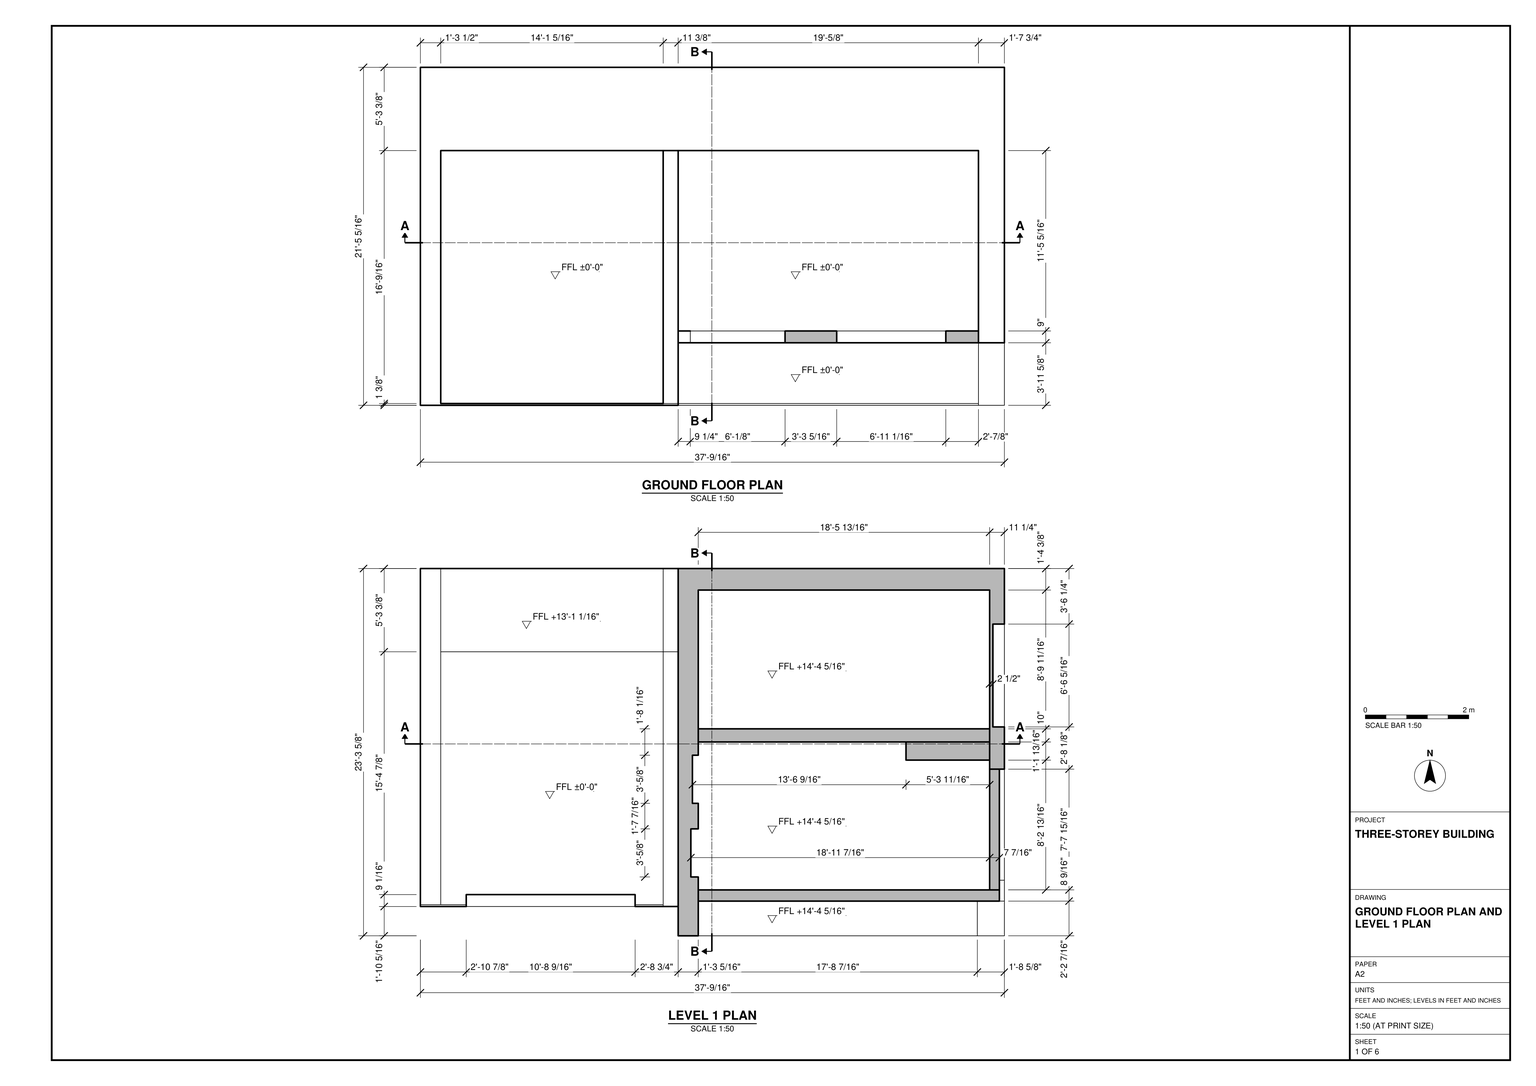
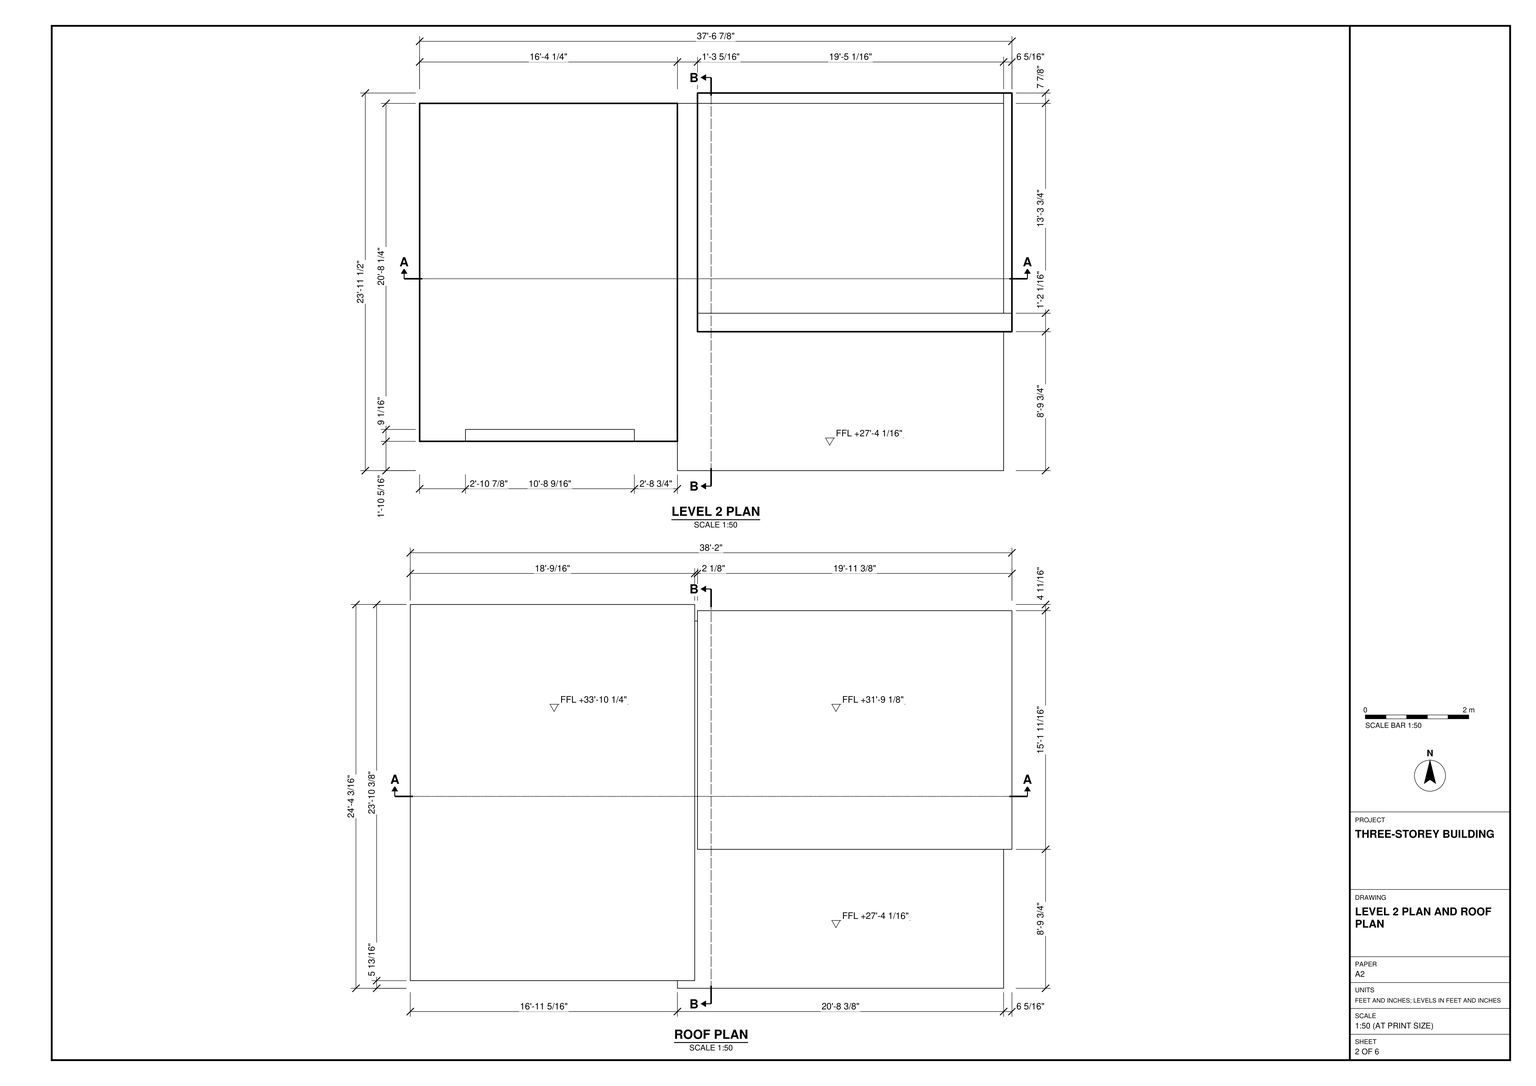
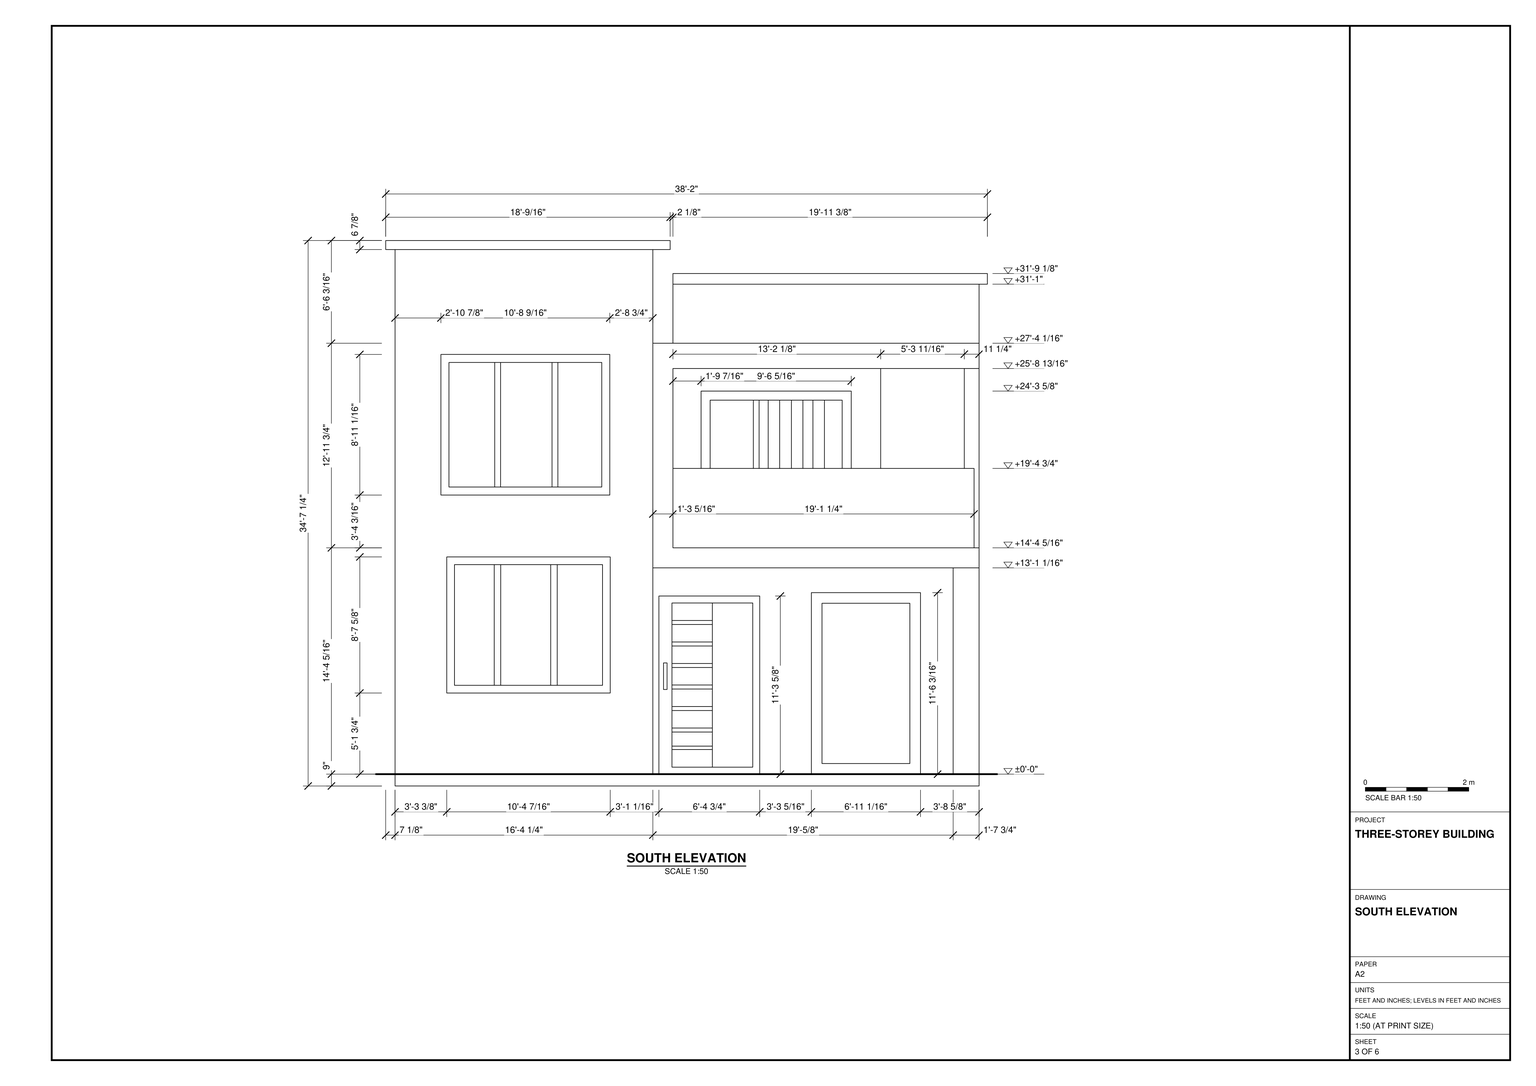
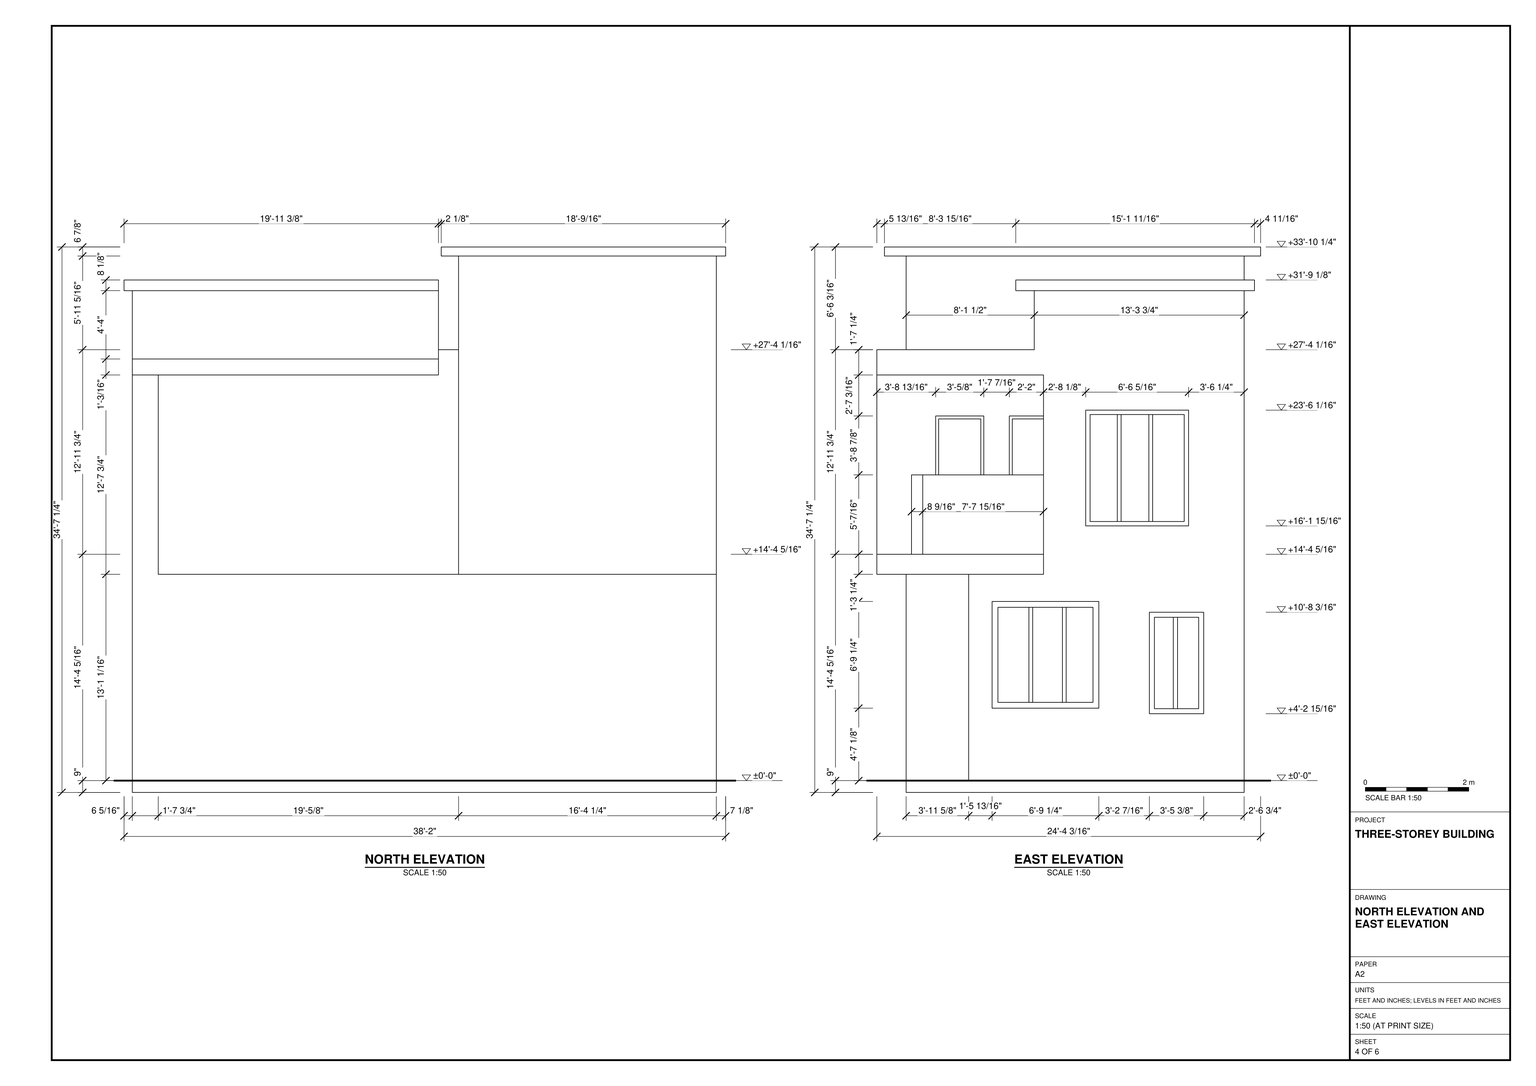
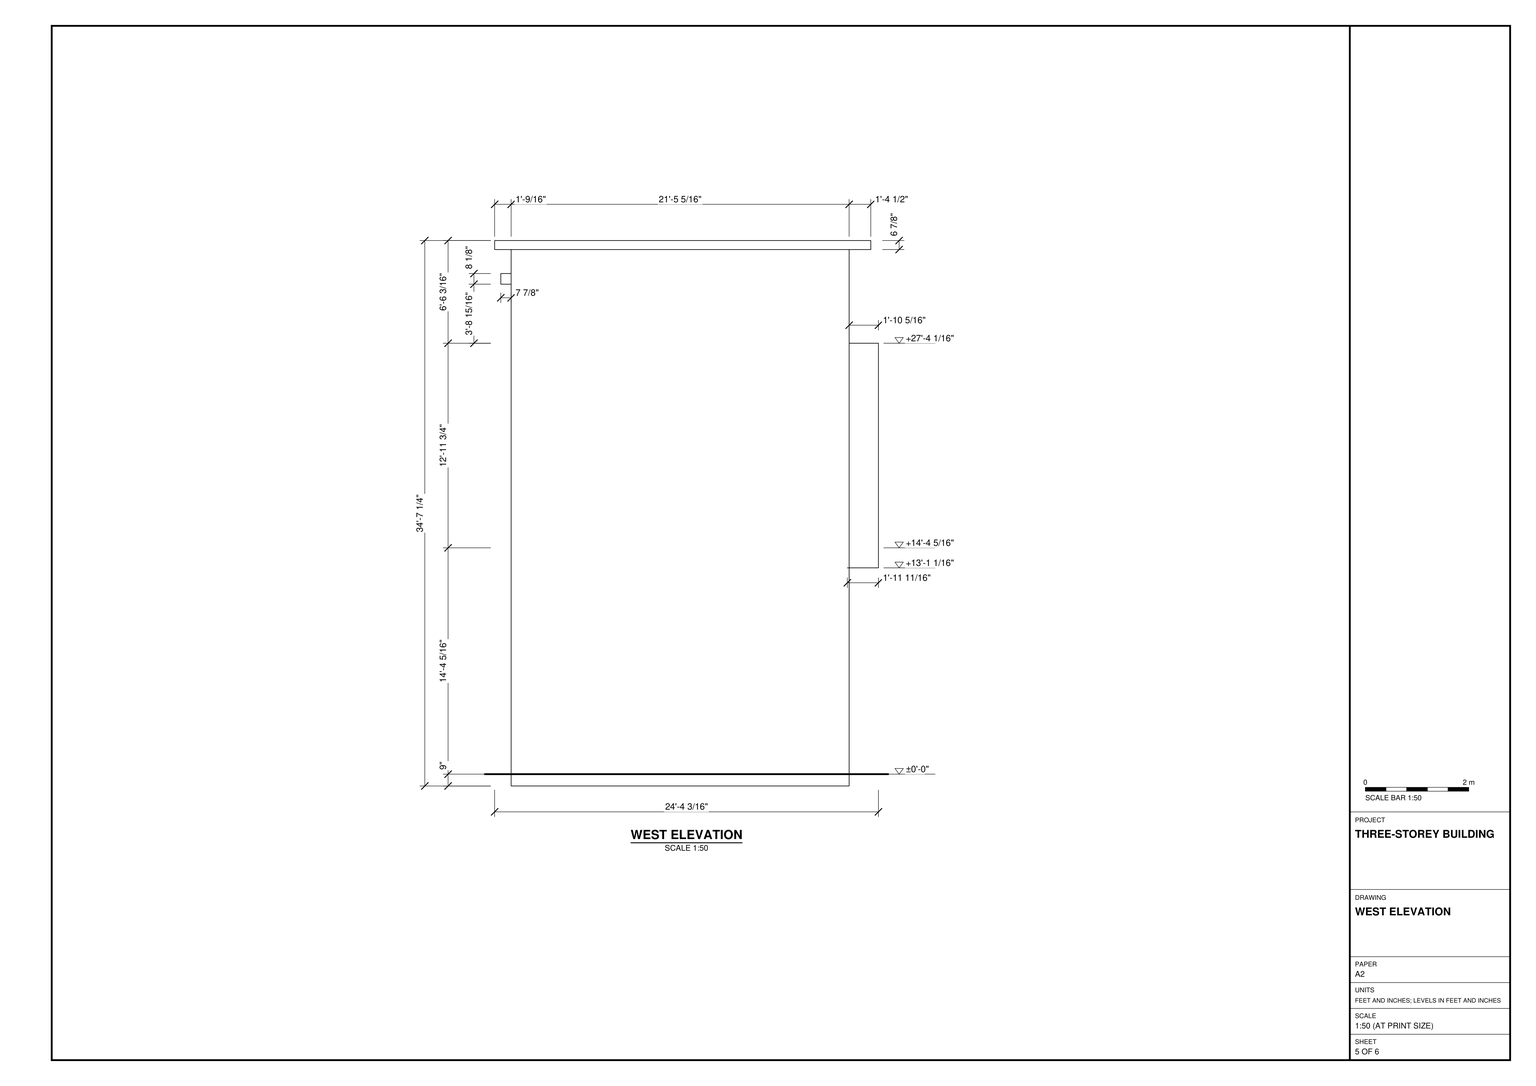
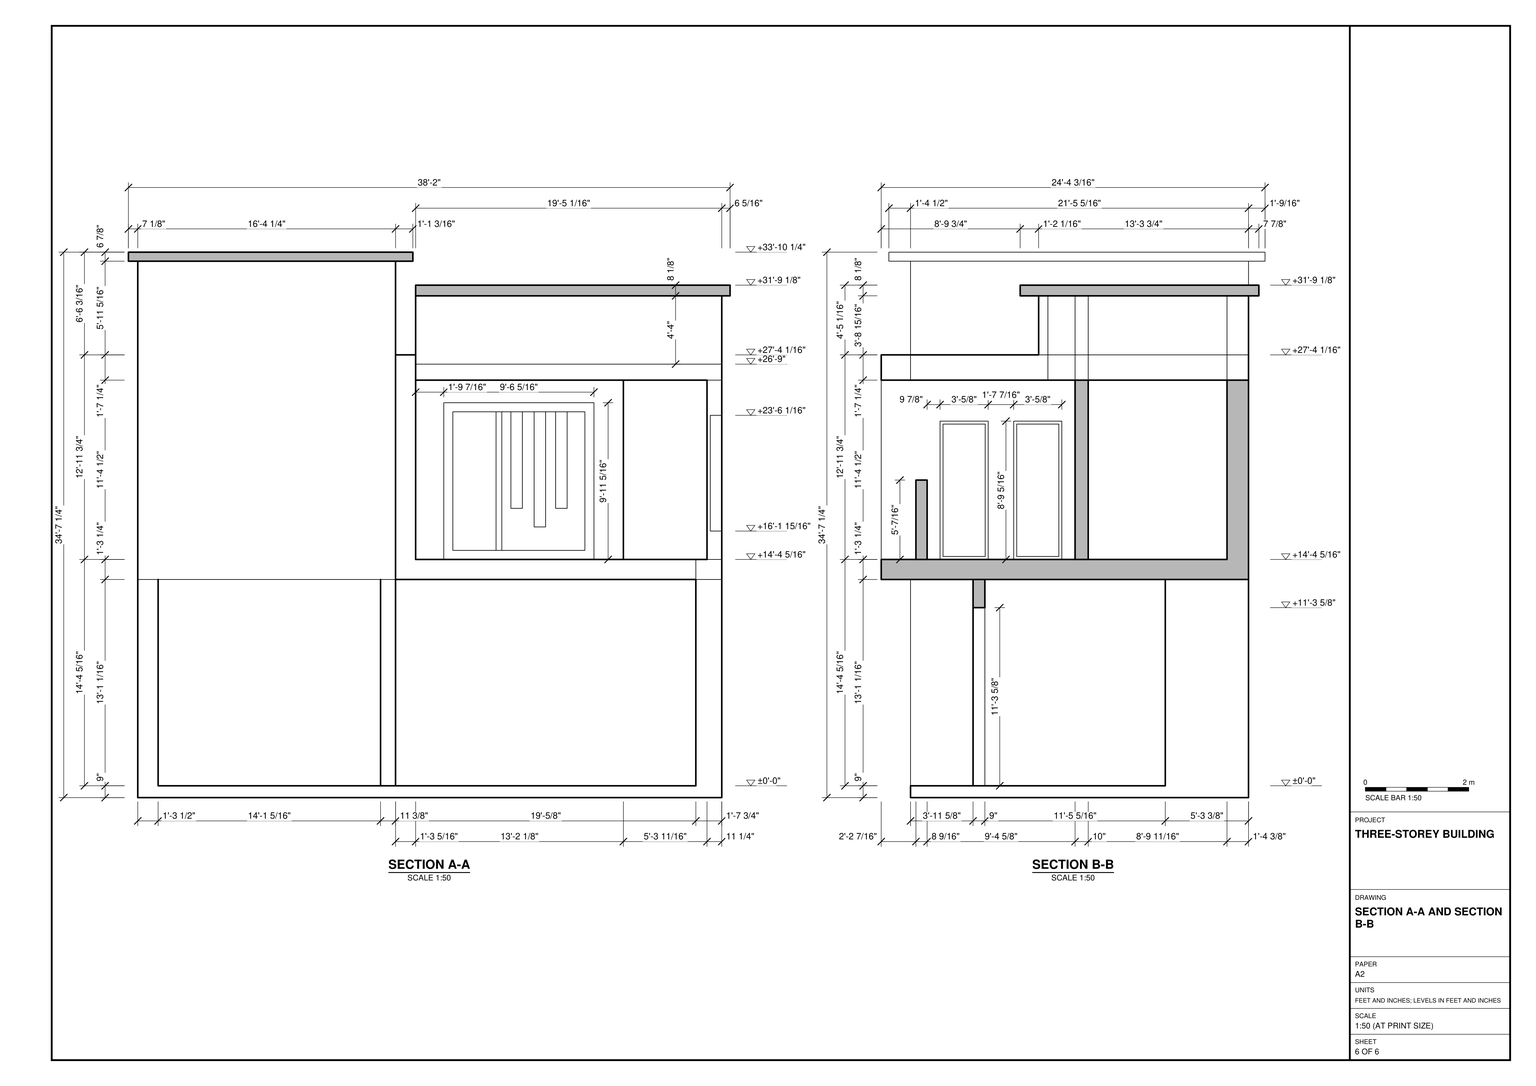
Build the three-storey building in SketchUp using task_files/diagram_01.pdf. Work in feet and inches. The overall model extents are 38'-2" along X, 24'-4 3/16" along Y and 34'-7 1/4" along Z. Set the ground floor at ±0'-0", Level 1 at +14'-4 5/16" and Level 2 at +27'-4 1/16".

Lay out the two adjoining bays from the plans. Follow the wall thicknesses, returns and slab outlines at each level, keeping the area marked at ground-floor level on the Level 1 plan open above. Use the south elevation to place the stacked window units in the taller bay and the entrance door and adjacent tall opening in the other bay. Model the recessed balcony above the entrance, including its solid front and the framed opening behind it. Match the separate flat roof slabs to their respective footprints and heights, leaving the front part of Level 2 exposed as drawn. Include stairs, built-in joinery and main furniture only where shown.

Keep walls, slabs, roofs and each furniture or joinery piece in separate groups or components, and use components for repeated parts. Decor and loose items may be any suitable library components. Save one SketchUp model as output_files/three_storey_building_with_recessed_balcony.skp.

# SketchUp Ruby script. Lengths in inches.
U = 1.inch
M = Sketchup.active_model
def pt(a) = Geom::Point3d.new(a.map { |v| v * U })
def face(e, loops, mat)
  f = e.add_face(loops[0].map { |a| pt(a) })
  loops[1..].each { |l| e.add_face(l.map { |a| pt(a) }).erase! }
  f.material = f.back_material = mat if mat
  f
end
# faces: each face lists its corners as indices into pts; further lists are holes
def faces(e, pts, list, mat = nil) = list.each { |f| face(e, (f[0].is_a?(Array) ? f : [f]).map { |l| l.map { |i| pts[i] } }, mat) }
# xy, xz, yz: faces in a plane at the given z, y or x. An outline is a flat list of corners, or four numbers for a rectangle; further outlines are holes
def ring(l) = l.size == 4 ? [[l[0], l[1]], [l[2], l[1]], [l[2], l[3]], [l[0], l[3]]] : l.each_slice(2).to_a
def flat(e, list, mat, &to3) = list.each { |f| face(e, (f[0].is_a?(Array) ? f : [f]).map { |l| ring(l).map { |u, v| to3.(u, v) } }, mat) }
def xy(e, z, list, mat = nil) = flat(e, list, mat) { |x, y| [x, y, z] }
def xz(e, y, list, mat = nil) = flat(e, list, mat) { |x, z| [x, y, z] }
def yz(e, x, list, mat = nil) = flat(e, list, mat) { |y, z| [x, y, z] }
def lines(e, pts, list) = list.each { |a, b| e.add_line(pt(pts[a]), pt(pts[b])) }
# prism: a flat outline (further loops are holes) pulled along v
def prism(e, loops, v, mat = nil)
  f = face(e, loops, mat); d = Geom::Vector3d.new(v.map { |x| x * U })
  f.pushpull(f.normal.samedirection?(d) ? d.length : -d.length)
end
def box(e, o, s, mat = nil) = prism(e, [[o, [o[0] + s[0], o[1], o[2]], [o[0] + s[0], o[1] + s[1], o[2]], [o[0], o[1] + s[1], o[2]]]], [0, 0, s[2]], mat)
def at(x, y, z, deg = 0) = Geom::Transformation.translation(pt([x, y, z])) * Geom::Transformation.rotation(ORIGIN, Z_AXIS, deg.degrees)
def axes(o, x, y, z) = Geom::Transformation.new([*x, 0, *y, 0, *z, 0, *pt(o).to_a, 1])
def part(name) = M.definitions.add(name)
# library, detail: a bought-in or finely detailed component or shape, given as its bounding box
def library(name, o, s) = part(name).tap { |d| box(d.entities, o, s) }
def detail(e, o, s) = box(e.add_group.entities, o, s)
def put(e, d, t, mat = nil) = e.add_instance(d, t).tap { |i| i.material = mat if mat }
def group(e, t, mat = nil) = e.add_group.tap { |g| g.transformation = t; g.material = mat if mat }.entities
root = M.entities
M.materials.add("[Formica Beige]").color = [211, 187, 149]
M.materials.add("[Formica Laminate Dark]").color = [50, 53, 60]
M.materials.add("[Formica Laminate Light]").color = [213, 189, 164]
M.materials.add("[Formica Speckled Grey]").color = [56, 62, 66]
M.materials.add("[Formica Speckled Grey]1").color = [94, 105, 111]
M.materials.add("[Quartz Light Brown]").color = [199, 184, 152]
M.materials.add("[Translucent Glass Gray]").color = [128, 128, 128]
M.materials["[Translucent Glass Gray]"].alpha = 0.5
M.materials.add("[Translucent Glass Safety]").color = [204, 235, 244]
M.materials["[Translucent Glass Safety]"].alpha = 0.5
M.materials.add("[Wood Floor Dark]").color = [153, 94, 42]
M.materials.add("[Wood Floor Light]").color = [204, 176, 127]
M.materials.add("[Wood Floor Parquet]").color = [81, 50, 21]
M.materials.add("[Wood Floor]").color = [91, 62, 36]
M.materials.add("[Wood Veneer 01]").color = [84, 49, 25]
M.materials.add("[Wood Veneer 01]1").color = [120, 70, 37]
xy(root,0,[[7.125,22.3125,451.7,279.61]])
xy(root,9,[[203.35,22.3125,431.96,23.68],[431.96,22.3125,451.7,69.91],[22.61,23.68,191.94,216.24],[191.94,23.68,203.35,216.24],[203.35,23.68,431.96,69.91],
  [203.35,69.91,212.59,78.9],[212.59,69.91,284.72,78.9],[284.72,69.91,324.04,78.9],[324.04,69.91,407.1,78.9],[407.1,69.91,431.96,78.9],
  [203.35,78.9,431.96,216.24]])
xy(root,144.625,[[212.59,69.91,284.72,78.9]])
xy(root,147.1875,[[324.04,69.91,407.1,78.9]])
xy(root,166.0625,[[203.35,0,451.7,69.91],[203.35,69.91,431.96,78.9],[431.96,69.91,451.7,78.9],[203.35,78.9,431.96,216.24],[22.61,216.24,191.94,279.61],
  [191.94,216.24,203.35,279.61],[203.35,216.24,431.96,279.61]])
xy(root,181.3125,[[218.65,0,431.09,26.41],[431.09,0,451.7,26.41],[218.65,26.41,431.09,34.95],[431.09,26.41,447.9,34.95],[447.9,26.41,451.7,42.31],
  [218.65,34.95,440.46,34.95,440.46,133.76,376.8,133.76,376.8,147.57,218.65,147.57,218.65,137.48,214.21,137.48,214.21,100.85,218.65,100.85,218.65,81.42,213.02,81.42,213.02,44.79,218.65,44.79],[440.46,34.95,447.9,126.88],[447.9,42.31,451.7,126.88],[376.8,133.76,431.96,147.57],[431.96,133.76,440.46,147.57],
  [218.65,147.57,440.46,157.57],[218.65,157.57,440.46,263.23]])
xy(root,202.92,[[442.95,159.01,451.7,237.33]])
xy(root,221.48,[[42.02,22.3125,170.58,31.375]])
xy(root,241.75,[[218.65,26.41,447.9,34.95],[440.46,34.95,447.9,126.88]],"[Translucent Glass Safety]")
xy(root,286.625,[[213.02,44.79,218.65,81.42],[214.21,100.85,218.65,137.48]])
xy(root,291.04,[[442.95,159.01,451.7,237.33]])
xy(root,317.8125,[[218.65,0,218.65,147.57,376.8,147.57,376.8,133.76,440.46,133.76,440.46,0],[440.46,0,451.7,126.88],[376.8,133.76,440.46,147.57],[218.65,147.57,440.46,157.57],[218.65,157.57,440.46,263.23],
  [218.65,263.23,440.46,279.61]])
xy(root,328.54,[[42.02,22.3125,170.58,31.375]])
xy(root,337.0625,[[203.35,0,451.7,0,451.7,119.84,218.65,119.84,218.65,279.61,203.35,279.61]])
xy(root,382,[[218.65,105.77,458.01,119.84],[218.65,119.84,451.7,279.61],[451.7,119.84,458.01,287.48],[218.65,279.61,451.7,287.48]])
xy(root,390.125,[[218.65,105.77,458.01,287.48]])
xy(root,408.375,[[7.125,22.3125,203.35,279.61],[7.125,279.61,203.35,292.17]])
xy(root,408.375,[[0,5.8125,216.53,22.3125],[0,22.3125,7.125,292.17],[203.35,22.3125,216.53,292.17]],"[Formica Speckled Grey]1")
xy(root,415.25,[[0,5.8125,216.53,292.17]])
xz(root,0,[[203.35,166.0625,451.7,166.0625,451.7,181.3125,218.65,181.3125,218.65,317.8125,451.7,317.8125,451.7,337.0625,203.35,337.0625]])
xz(root,5.8125,[[0,408.375,216.53,415.25]])
xz(root,22.3125,[[[7.125,0,451.7,0,451.7,9,203.35,9,203.35,408.375,7.125,408.375],[42.02,221.48,170.58,328.54],[46.48,70.76,170.92,174.38]]])
xz(root,22.3125,[[[46.48,70.76,170.92,174.38],[52.35,76.63,165.05,168.52]],[82.61,76.63,87.56,168.52],[125.61,76.63,130.56,168.52]],"[Formica Speckled Grey]")
xz(root,22.3125,[[52.35,76.63,82.61,168.52],[87.56,76.63,125.61,168.52],[130.56,76.63,165.05,168.52]],"[Translucent Glass Safety]")
xz(root,23.68,[[22.61,9,191.94,166.0625]])
xz(root,26.41,[[218.65,181.3125,447.9,241.75]],"[Translucent Glass Safety]")
xz(root,31.375,[[[42.02,221.48,170.58,328.54],[48.14,227.6,164.46,322.42]],[82.98,227.6,87.4375,322.42],[126.6,227.6,131.0625,322.42]],"[Formica Speckled Grey]")
xz(root,31.375,[[48.14,227.6,82.98,322.42],[87.4375,227.6,126.6,322.42],[131.0625,227.6,164.46,322.42]],"[Translucent Glass Safety]")
xz(root,34.95,[[431.09,181.3125,440.46,241.75],[440.46,181.3125,447.9,241.75]])
xz(root,34.95,[[218.65,181.3125,431.09,241.75]],"[Translucent Glass Safety]")
xz(root,44.79,[[213.02,181.3125,218.65,286.625]])
xz(root,69.91,[[203.35,9,207.97,9,207.97,144.625,284.72,144.625,284.72,9,324.04,9,324.04,147.1875,407.1,147.1875,407.1,9,431.96,9,431.96,166.0625,203.35,166.0625],[431.96,9,451.7,166.0625]])
xz(root,69.91,[[211.49,73.44,214.17,93.69]],"[Formica Beige]")
xz(root,69.91,[[217.9,27.75,248.65,30.33],[217.9,41.0625,248.65,44.12],[217.9,57.4375,248.65,60.5],[217.9,73.8125,248.65,76.87],[217.9,90.1875,248.65,93.25],
  [217.9,106.5625,248.65,109.62],[217.9,122.9375,248.65,126]],"[Quartz Light Brown]")
xz(root,69.91,[[332.125,17.09,399.01,139.1]],"[Translucent Glass Gray]")
xz(root,69.91,[[248.65,14.3125,279.41,139.3125]],"[Translucent Glass Safety]")
xz(root,69.91,[[217.9,14.3125,248.65,27.75],[217.9,30.33,248.65,41.0625],[217.9,44.12,248.65,57.4375],[217.9,60.5,248.65,73.8125],[217.9,76.87,248.65,90.1875],
  [217.9,93.25,248.65,106.5625],[217.9,109.62,248.65,122.9375],[217.9,126,248.65,139.3125]],"[Wood Floor Dark]")
xz(root,69.91,[[[207.97,9,284.72,144.625],[217.9,14.3125,279.41,139.3125],[211.49,73.44,214.17,93.69]]],"[Wood Floor Parquet]")
xz(root,69.91,[[[324.04,9,407.1,147.1875],[332.125,17.09,399.01,139.1]]],"[Wood Floor]")
xz(root,78.9,[[203.35,9,203.35,166.0625,431.96,166.0625,431.96,9,407.1,9,407.1,147.1875,324.04,147.1875,324.04,9,284.72,9,284.72,144.625,212.59,144.625,212.59,9]])
xz(root,81.42,[[213.02,181.3125,218.65,286.625]])
xz(root,100.85,[[214.21,181.3125,218.65,286.625]])
xz(root,105.77,[[218.65,382,458.01,390.125]])
xz(root,119.84,[[218.65,337.0625,451.7,382]])
xz(root,126.88,[[440.46,181.3125,447.9,241.75],[447.9,181.3125,451.7,181.3125,451.7,317.8125,440.46,317.8125,440.46,241.75,447.9,241.75]])
xz(root,133.76,[[376.8,181.3125,440.46,317.8125]])
xz(root,137.48,[[214.21,181.3125,218.65,286.625]])
xz(root,147.57,[[218.65,181.3125,240.07,181.3125,240.07,300.625,354.38,300.625,354.38,181.3125,376.8,181.3125,376.8,317.8125,218.65,317.8125],[376.8,181.3125,440.46,317.8125]])
xz(root,147.57,[[284.24,188.21,347.48,188.21,347.48,293.72,333.98,293.72,333.98,220.22,325.23,220.22,325.23,293.72,317.6,293.72,317.6,206.07,308.85,206.07,308.85,293.72,299.91,293.72,299.91,220.22,291.16,220.22,291.16,293.72,284.24,293.72]],"[Wood Floor Light]")
xz(root,147.57,[[246.97,188.21,279.86,293.72]],"[Wood Floor Parquet]")
xz(root,147.57,[[[240.07,181.3125,354.38,300.625],[246.97,188.21,347.48,293.72]],[279.86,188.21,284.24,293.72],[308.85,206.07,317.6,293.72],[291.16,220.22,299.91,293.72],[325.23,220.22,333.98,293.72]],"[Wood Veneer 01]")
xz(root,157.57,[[218.65,181.3125,440.46,317.8125]])
xz(root,159.01,[[442.95,202.92,451.7,291.04]])
xz(root,216.24,[[22.61,9,191.94,166.0625],[191.94,9,203.35,166.0625],[203.35,9,431.96,166.0625]])
xz(root,237.33,[[442.95,202.92,451.7,291.04]])
xz(root,263.23,[[218.65,181.3125,440.46,317.8125]])
xz(root,279.61,[[7.125,0,7.125,166.0625,431.96,166.0625,431.96,317.8125,451.7,317.8125,451.7,0],[7.125,166.0625,203.35,408.375],[203.35,166.0625,203.35,337.0625,218.65,337.0625,218.65,317.8125,431.96,317.8125,431.96,166.0625],[218.65,317.8125,451.7,330],[218.65,330,451.7,382]])
xz(root,287.48,[[218.65,382,458.01,390.125]])
xz(root,292.17,[[0,408.375,216.53,415.25]])
yz(root,0,[[5.8125,408.375,292.17,415.25]])
yz(root,7.125,[[22.3125,0,279.61,408.375]])
yz(root,22.61,[[23.68,9,216.24,166.0625]])
yz(root,42.02,[[22.3125,221.48,31.375,328.54]])
yz(root,170.58,[[22.3125,221.48,31.375,328.54]])
yz(root,191.94,[[23.68,9,216.24,166.0625]])
yz(root,203.35,[[22.3125,9,69.91,166.0625],[69.91,9,78.9,166.0625],[78.9,9,216.24,166.0625],[0,166.0625,22.3125,337.0625],[22.3125,166.0625,279.61,337.0625],
  [22.3125,337.0625,279.61,408.375]])
yz(root,213.02,[[47.0625,183.58,79.15,284.35]],"[Formica Laminate Light]")
yz(root,213.02,[[[44.79,181.3125,81.42,286.625],[47.0625,183.58,79.15,284.35]]],"[Wood Floor Parquet]")
yz(root,214.21,[[103.125,183.58,135.21,284.35]],"[Formica Laminate Light]")
yz(root,214.21,[[[100.85,181.3125,137.48,286.625],[103.125,183.58,135.21,284.35]]],"[Wood Veneer 01]1")
yz(root,216.53,[[5.8125,408.375,292.17,415.25]])
yz(root,218.65,[[0,181.3125,26.41,181.3125,26.41,241.75,34.95,241.75,34.95,181.3125,44.79,181.3125,44.79,286.625,81.42,286.625,81.42,181.3125,100.85,181.3125,100.85,286.625,137.48,286.625,137.48,181.3125,147.57,181.3125,147.57,317.8125,0,317.8125],[26.41,181.3125,34.95,241.75],[147.57,181.3125,157.57,317.8125],[157.57,181.3125,263.23,317.8125],[126.88,317.8125,147.57,337.0625],
  [147.57,317.8125,157.57,337.0625],[157.57,317.8125,263.23,337.0625],[263.23,317.8125,279.61,337.0625],[119.84,337.0625,126.88,382],[126.88,337.0625,147.57,382],
  [147.57,337.0625,157.57,382],[157.57,337.0625,263.23,382],[263.23,337.0625,279.61,382],[105.77,382,126.88,390.125],[126.88,382,147.57,390.125],
  [147.57,382,157.57,390.125],[157.57,382,263.23,390.125],[263.23,382,287.48,390.125]])
yz(root,284.72,[[69.91,9,78.9,144.625]])
yz(root,324.04,[[69.91,9,78.9,147.1875]])
yz(root,376.8,[[133.76,181.3125,147.57,317.8125]])
yz(root,407.1,[[69.91,9,78.9,147.1875]])
yz(root,431.96,[[69.91,9,78.9,166.0625],[78.9,9,216.24,166.0625]])
yz(root,440.46,[[126.88,181.3125,133.76,317.8125],[133.76,181.3125,147.57,317.8125],[147.57,181.3125,157.57,317.8125],[157.57,181.3125,263.23,317.8125]])
yz(root,440.46,[[34.95,181.3125,126.88,241.75]],"[Translucent Glass Safety]")
yz(root,442.95,[[[159.01,202.92,237.33,291.04],[162.34,206.25,233.99,287.71]],[183.07,206.25,185.95,287.71],[207.09,206.25,209.97,287.71]],"[Formica Laminate Dark]")
yz(root,442.95,[[162.34,206.25,183.07,287.71],[185.95,206.25,207.09,287.71],[209.97,206.25,233.99,287.71]],"[Translucent Glass Gray]")
yz(root,447.9,[[26.41,181.3125,34.95,241.75],[34.95,181.3125,126.88,241.75]],"[Translucent Glass Safety]")
yz(root,451.7,[[[22.3125,0,279.61,0,279.61,382,119.84,382,119.84,337.0625,0,337.0625,0,317.8125,126.88,317.8125,126.88,166.0625,69.91,166.0625,69.91,9,22.3125,9],[159.01,202.92,237.33,291.04],[87.75,64.14,169,145.39],[207.47,59.93,248.84,137.18]],[0,166.0625,126.88,181.3125]])
yz(root,451.7,[[[207.47,59.93,248.84,137.18],[211.3,63.77,245.01,133.35]],[225.69,63.77,228.93,133.35],[[87.75,64.14,169,145.39],[92.1875,68.58,164.56,140.95]],[115.79,68.58,118.64,140.95],[141.29,68.58,144.14,140.95]],"[Formica Laminate Dark]")
yz(root,451.7,[[211.3,63.77,225.69,133.35],[228.93,63.77,245.01,133.35],[92.1875,68.58,115.79,140.95],[118.64,68.58,141.29,140.95],[144.14,68.58,164.56,140.95]],"[Translucent Glass Gray]")
yz(root,458.01,[[105.77,382,287.48,390.125]])
p = [[7.125,22.3125,166.0625],[7.125,23.68,166.0625],[431.96,147.57,166.0625],[431.96,147.57,181.3125],[431.96,216.24,166.0625],[431.96,216.24,181.3125],
  [451.7,147.57,166.0625],[440.46,147.57,181.3125],[451.7,147.57,181.3125],[191.94,23.68,166.0625],[191.94,22.3125,166.0625],[22.61,23.68,166.0625],
  [440.46,157.57,317.8125],[451.7,157.57,317.8125],[440.46,133.76,317.8125],[451.7,133.76,317.8125],[440.46,147.57,317.8125],[451.7,147.57,317.8125]]
lines(root,p,[[0,1],[2,3],[4,5],[2,6],[7,8],[9,10],[11,1],[12,13],[14,15],[16,17]])
